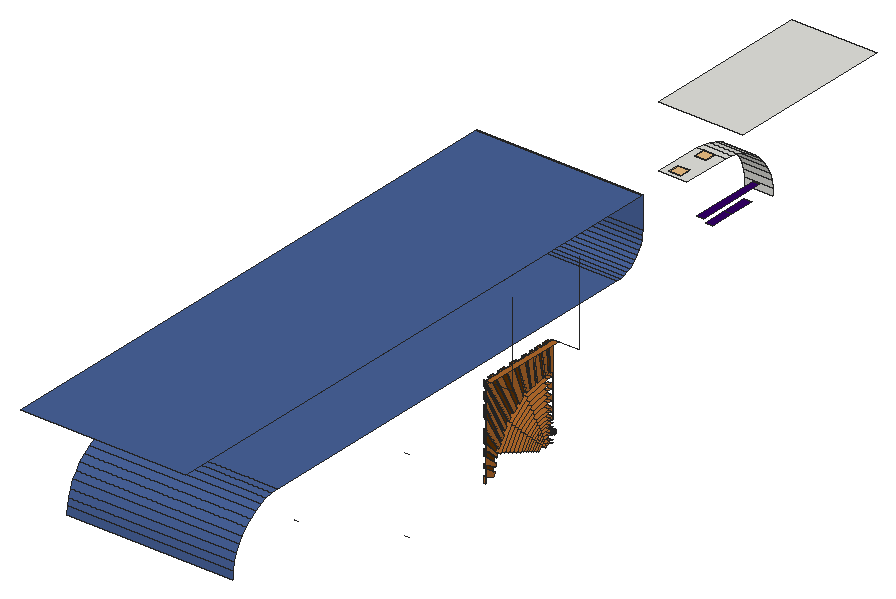
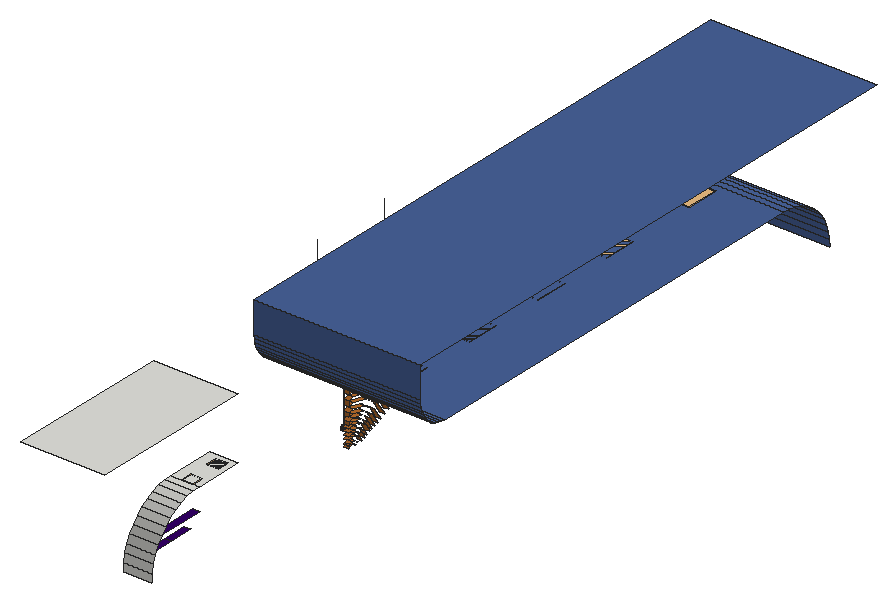
# SketchUp Ruby script. Lengths in inches.
U = 1.inch
M = Sketchup.active_model
def pt(a) = Geom::Point3d.new(a.map { |v| v * U })
def face(e, loops, mat)
  f = e.add_face(loops[0].map { |a| pt(a) })
  loops[1..].each { |l| e.add_face(l.map { |a| pt(a) }).erase! }
  f.material = f.back_material = mat if mat
  f
end
# faces: each face lists its corners as indices into pts; further lists are holes
def faces(e, pts, list, mat = nil) = list.each { |f| face(e, (f[0].is_a?(Array) ? f : [f]).map { |l| l.map { |i| pts[i] } }, mat) }
# xy, xz, yz: faces in a plane at the given z, y or x. An outline is a flat list of corners, or four numbers for a rectangle; further outlines are holes
def ring(l) = l.size == 4 ? [[l[0], l[1]], [l[2], l[1]], [l[2], l[3]], [l[0], l[3]]] : l.each_slice(2).to_a
def flat(e, list, mat, &to3) = list.each { |f| face(e, (f[0].is_a?(Array) ? f : [f]).map { |l| ring(l).map { |u, v| to3.(u, v) } }, mat) }
def xy(e, z, list, mat = nil) = flat(e, list, mat) { |x, y| [x, y, z] }
def xz(e, y, list, mat = nil) = flat(e, list, mat) { |x, z| [x, y, z] }
def yz(e, x, list, mat = nil) = flat(e, list, mat) { |y, z| [x, y, z] }
def lines(e, pts, list) = list.each { |a, b| e.add_line(pt(pts[a]), pt(pts[b])) }
# prism: a flat outline (further loops are holes) pulled along v
def prism(e, loops, v, mat = nil)
  f = face(e, loops, mat); d = Geom::Vector3d.new(v.map { |x| x * U })
  f.pushpull(f.normal.samedirection?(d) ? d.length : -d.length)
end
def box(e, o, s, mat = nil) = prism(e, [[o, [o[0] + s[0], o[1], o[2]], [o[0] + s[0], o[1] + s[1], o[2]], [o[0], o[1] + s[1], o[2]]]], [0, 0, s[2]], mat)
def at(x, y, z, deg = 0) = Geom::Transformation.translation(pt([x, y, z])) * Geom::Transformation.rotation(ORIGIN, Z_AXIS, deg.degrees)
def axes(o, x, y, z) = Geom::Transformation.new([*x, 0, *y, 0, *z, 0, *pt(o).to_a, 1])
def part(name) = M.definitions.add(name)
# library, detail: a bought-in or finely detailed component or shape, given as its bounding box
def library(name, o, s) = part(name).tap { |d| box(d.entities, o, s) }
def detail(e, o, s) = box(e.add_group.entities, o, s)
def put(e, d, t, mat = nil) = e.add_instance(d, t).tap { |i| i.material = mat if mat }
def group(e, t, mat = nil) = e.add_group.tap { |g| g.transformation = t; g.material = mat if mat }.entities
root = M.entities
M.materials.add("[Color C08]").color = [102, 51, 0]
M.materials.add("[Color J08]").color = [51, 0, 102]
M.materials.add("[Formica Blue]").color = [71, 97, 152]
M.materials.add("[Wood Bamboo]").color = [177, 105, 43]
c1 = part("Recessed light")
detail(c1.entities,[0,0,0],[14.08,14.08,3])
c2 = part("Recessed light \#1")
detail(c2.entities,[0,0,0],[4.875,4.875,1.1875])
xy(root,196.65,[[182,311.38,185,321.81],[182,321.81,185,332.23]],"[Color J08]")
xy(root,201.38,[[182,306.65,185,336.96]],"[Color J08]")
xy(root,209.98,[[205.625,165.13,206.625,167.88],[205.625,170.69,206.625,173.92],[205.625,177.27,206.625,180.4],[205.625,183.39,206.625,185.625],[205.625,187.86,206.625,189.13],
  [205.625,190.73,206.625,192.46],[205.625,192.46,206.625,193.08],[205.625,195.09,206.625,196.125],[205.625,196.125,206.625,197.55]],"[Wood Bamboo]")
xy(root,210,[[206.625,162.98,209,198.98]],"[Wood Bamboo]")
xy(root,219.12,[[137.625,49.45,208.5625,230.99]],"[Formica Blue]")
xy(root,219.28,[[173,297.87,185,318.3125]])
xy(root,246,[[173,297.87,209,369.14]])
xy(root,246,[[137.625,0.14,208.5625,244.43]],"[Formica Blue]")
xz(root,163,[[205.625,170.21,206.625,173.125],[205.625,176.04,206.625,177.78],[205.625,180.75,206.625,183.41],[205.625,185.93,206.625,191.12],[205.625,195.86,206.625,200.46],
  [205.625,202.96,206.625,205.25],[205.625,207.6,206.625,209.97]],"[Wood Bamboo]")
xz(root,198.97,[[204.625,179.23,206.625,180.69],[204.625,182.32,206.625,184.08],[204.625,186.37,206.625,188.67],[204.625,190.87,206.625,193.18],[204.625,195.77,206.625,197.62]],"[Wood Bamboo]")
xz(root,244.43,[[137.625,232.56,208.5625,246]],"[Formica Blue]")
yz(root,205.625,[[167.88,172.94,163,176.04,163,177.78,168.17,174.44],[168.49,176.05,163,180.75,163,183.41,168.83,177.79],[169.125,179.3125,163,185.93,163,191.12,170.04,180.72],[170.96,182.13,163,195.86,163,200.46,171.63,183.15],[172.58,184.61,163,202.96,163,205.25,173.46,185.97],
  [174.375,187.37,163,207.6,163,209.97,175.42,188.97],[176.54,189.75,165.13,209.98,167.88,209.98,178.08,190.8125],[179.64,191.9,170.69,209.98,173.92,209.98,181.39,193.12],[183.14,194.33,177.27,209.98,180.4,209.98,184.88,195.55],[186.57,195.93,183.39,209.98,185.625,209.98,187.86,196.22],
  [189.29,196.54,187.86,209.98,189.13,209.98,191.14,196.96,190.73,196.87],[193.12,197.41,190.73,209.98,193.08,209.98,195.09,197.86,193.65,197.53],[197.98,197.78,197.55,197.86,196.125,198.09,195.09,209.98,197.55,209.98]],"[Color C08]")
yz(root,206.625,[[163,170.21,162.98,170.22,162.98,176.05,163,176.04],[167.48,170.9,163,173.125,163,176.04,167.88,172.94],[168.17,174.44,163,177.78,163,180.75,168.49,176.05],[163,176.04,162.98,176.05,162.98,177.79,163,177.78],[163,177.78,162.98,177.79,162.98,180.77,163,180.75],
  [168.83,177.79,163,183.41,163,185.93,169.125,179.3125],[198.97,179.23,198.97,180.69,198.98,180.6875,198.98,179.23],[198.98,180.6875,198.97,180.69,198.97,182.32,198.98,182.32],[170.04,180.72,163,191.12,163,195.86,170.96,182.13],[163,180.75,162.98,180.77,162.98,183.42,163,183.41],
  [198.97,182.32,198.98,184.08],[171.63,183.15,163,200.46,163,202.96,172.58,184.61],[163,183.41,162.98,183.42,162.98,210,163,209.97],[198.97,184.08,198.98,186.37],[173.46,185.97,163,205.25,163,207.6,174.375,187.37],
  [198.97,186.37,198.97,188.67,198.98,188.66,198.98,186.37],[198.98,188.66,198.97,188.67,198.97,190.87,198.98,190.86],[175.42,188.97,163,209.97,163,209.98,165.13,209.98,176.54,189.75],[178.08,190.8125,167.88,209.98,170.69,209.98,179.64,191.9],[198.98,190.86,198.97,190.87,198.97,193.18,198.98,193.18],
  [181.39,193.12,173.92,209.98,177.27,209.98,183.14,194.33],[198.97,193.18,198.98,195.77],[184.88,195.55,180.4,209.98,183.39,209.98,186.57,195.93],[198.97,195.77,198.98,197.62],[187.86,196.22,185.625,209.98,187.86,209.98,189.29,196.54],
  [191.14,196.96,189.13,209.98,190.73,209.98,193.12,197.41,192.46,197.26,191.56,197.06],[198.97,197.62,197.98,197.78,197.55,209.98,198.97,209.98],[198.97,197.62,198.98,199.86],[195.09,197.86,193.08,209.98,195.09,209.98,196.125,198.09],[198.97,199.86,198.97,209.98,197.55,209.98,197.55,210,198.98,210,198.98,199.86],
  [163,209.97,162.98,210,187.85,210,187.86,209.98,163,209.98],[187.86,209.98,187.85,210,189.125,210,189.13,209.98],[189.13,209.98,189.125,210,190.72,210,190.73,209.98],[190.73,209.98,190.72,210,192.46,210,192.46,209.98],[192.46,209.98,195.09,210],
  [195.09,209.98,196.125,210],[196.125,209.98,197.55,210]],"[Wood Bamboo]")
p = [[206.625,195.85,170.66],[206.625,194.93,170.03],[204.625,194.93,170.03],[204.625,195.85,170.66],[206.625,198.98,170.15],[206.625,198.03,170.73],
  [204.625,198.03,170.73],[204.625,198.98,170.15],[206.625,192.8,172.09],[206.625,191.57,170.21],[204.625,191.57,170.21],[204.625,192.8,172.09],
  [206.625,190.3,170.73],[206.625,191.8125,173.05],[204.625,191.8125,173.05],[204.625,190.3,170.73],[206.625,196.93,170.91],[204.625,196.93,170.91],
  [206.625,194.14,170.79],[206.625,195.4,171.67],[204.625,195.4,171.67],[204.625,194.14,170.79],[206.625,163,173.125],[206.625,167.48,170.9],
  [205.625,167.48,170.9],[205.625,163,173.125],[206.625,190.77,174.07],[206.625,188.94,171.27],[204.625,188.94,171.27],[204.625,190.77,174.07],
  [206.625,198.42,171.76],[206.625,198.98,171.41],[204.625,198.98,171.41],[204.625,198.42,171.76],[206.625,196.9,172.01],[204.625,196.9,172.01],
  [206.625,187.43,171.89],[206.625,189.59,175.21],[204.625,189.59,175.21],[204.625,187.43,171.89],[206.625,194.65,173.38],[204.625,194.65,173.38],
  [206.625,188.6875,176.09],[206.625,186.26,172.36],[204.625,186.26,172.36],[204.625,188.6875,176.09],[206.625,167.88,172.94],[206.625,163,176.04],
  [205.625,163,176.04],[205.625,167.88,172.94],[206.625,184.9,172.92],[206.625,187.63,177.11],[204.625,187.63,177.11],[204.625,184.9,172.92],
  [206.625,194.09,174.64],[204.625,194.09,174.64],[206.625,196.84,173.875],[204.625,196.84,173.875],[206.625,186.46,178.25],[206.625,183.38,173.53],
  [204.625,183.38,173.53],[204.625,186.46,178.25],[206.625,198.98,173.52],[204.625,198.98,173.52],[206.625,193.51,175.97],[204.625,193.51,175.97],
  [206.625,181.74,174.2],[206.625,185.19,179.48],[204.625,185.19,179.48],[204.625,181.74,174.2],[206.625,163,177.78],[206.625,168.17,174.44],
  [205.625,168.17,174.44],[205.625,163,177.78],[206.625,196.8,175.25],[204.625,196.8,175.25],[206.625,198.98,174.89],[204.625,198.98,174.89],
  [206.625,183.54,181.09],[206.625,179.6,175.0625],[204.625,179.6,175.0625],[204.625,183.54,181.09],[206.625,192.85,177.47],[204.625,192.85,177.47],
  [206.625,177.47,175.93],[206.625,181.88,182.7],[204.625,181.88,182.7],[204.625,177.47,175.93],[206.625,168.49,176.05],[206.625,163,180.75],
  [205.625,163,180.75],[205.625,168.49,176.05],[206.625,196.76,176.71],[204.625,196.76,176.71],[206.625,192.34,178.63],[204.625,192.34,178.63],
  [206.625,198.98,176.35],[204.625,198.98,176.35],[206.625,180.29,184.24],[206.625,175.42,176.76],[204.625,175.42,176.76],[204.625,180.29,184.24],
  [206.625,191.75,179.97],[204.625,191.75,179.97],[206.625,196.71,178.34],[204.625,196.71,178.34],[206.625,173.26,177.64],[206.625,178.62,185.86],
  [204.625,178.62,185.86],[204.625,173.26,177.64],[206.625,163,183.41],[206.625,168.83,177.79],[205.625,168.83,177.79],[205.625,163,183.41],
  [206.625,198.98,177.97],[204.625,198.98,177.97],[206.625,191.08,181.47],[204.625,191.08,181.47],[206.625,176.76,187.67],[206.625,170.85,178.61],
  [204.625,170.85,178.61],[204.625,176.76,187.67],[206.625,196.67,179.61],[204.625,196.67,179.61],[206.625,198.97,179.23],[204.625,198.97,179.23],
  [206.625,169.125,179.3125],[206.625,163,185.93],[205.625,163,185.93],[205.625,169.125,179.3125],[204.625,169.125,179.3125],[205.625,170.04,180.72],
  [206.625,170.04,180.72],[206.625,170.96,182.13],[205.625,170.96,182.13],[205.625,171.63,183.15],[206.625,171.63,183.15],[206.625,172.58,184.61],
  [205.625,172.58,184.61],[205.625,173.46,185.97],[206.625,173.46,185.97],[206.625,174.375,187.37],[205.625,174.375,187.37],[205.625,175.42,188.97],
  [204.625,175.42,188.97],[206.625,190.375,183.09],[204.625,190.375,183.09],[206.625,196.63,181.08],[204.625,196.63,181.08],[206.625,163,191.12],
  [205.625,163,191.12],[206.625,198.97,180.69],[204.625,198.97,180.69],[206.625,189.44,185.2],[204.625,189.44,185.2],[206.625,196.58,182.71],
  [204.625,196.58,182.71],[206.625,163,195.86],[205.625,163,195.86],[206.625,198.97,182.32],[204.625,198.97,182.32],[206.625,188.51,187.31],
  [204.625,188.51,187.31],[206.625,196.53,184.48],[204.625,196.53,184.48],[206.625,163,200.46],[205.625,163,200.46],[206.625,198.97,184.08],
  [204.625,198.97,184.08],[206.625,187.62,189.33],[204.625,187.62,189.33],[206.625,163,202.96],[205.625,163,202.96],[206.625,196.46,186.78],
  [204.625,196.46,186.78],[206.625,186.68,191.46],[204.625,186.68,191.46],[206.625,163,205.25],[205.625,163,205.25],[206.625,198.97,186.37],
  [204.625,198.97,186.37],[206.625,196.39,189.09],[204.625,196.39,189.09],[206.625,163,207.6],[205.625,163,207.6],[206.625,185.63,193.84],
  [204.625,185.63,193.84],[206.625,198.97,188.67],[204.625,198.97,188.67],[206.625,163,209.97],[206.625,175.42,188.97],[205.625,163,209.97],
  [206.625,176.54,189.75],[205.625,176.54,189.75],[205.625,178.08,190.8125],[206.625,178.08,190.8125],[206.625,179.64,191.9],[205.625,179.64,191.9],
  [205.625,181.39,193.12],[206.625,181.39,193.12],[206.625,183.14,194.33],[205.625,183.14,194.33],[205.625,184.88,195.55],[204.625,184.88,195.55],
  [206.625,196.33,191.3],[204.625,196.33,191.3],[206.625,165.13,209.98],[205.625,165.13,209.98],[206.625,167.88,209.98],[205.625,167.88,209.98],
  [206.625,198.97,190.87],[204.625,198.97,190.87],[206.625,196.26,193.63],[204.625,196.26,193.63],[206.625,170.69,209.98],[205.625,170.69,209.98],
  [206.625,173.92,209.98],[205.625,173.92,209.98],[206.625,198.97,193.18],[204.625,198.97,193.18],[185,343.92,193.67],[185,343.7,197.02],
  [173,343.7,197.02],[173,343.92,193.67],[206.625,196.18,196.23],[204.625,196.18,196.23],[206.625,177.27,209.98],[205.625,177.27,209.98],
  [137.625,25.13,194.81],[137.625,25.34,197.98],[208.5625,25.34,197.98],[208.5625,25.13,194.81],[206.625,180.4,209.98],[206.625,184.88,195.55],
  [205.625,180.4,209.98],[206.625,186.57,195.93],[205.625,186.57,195.93],[205.625,187.86,196.22],[206.625,187.86,196.22],[206.625,189.29,196.54],
  [205.625,189.29,196.54],[205.625,190.73,196.87],[205.625,191.14,196.96],[206.625,191.14,196.96],[206.625,191.56,197.06],[206.625,192.46,197.26],
  [206.625,193.12,197.41],[205.625,193.12,197.41],[205.625,193.65,197.53],[205.625,195.09,197.86],[206.625,195.09,197.86],[206.625,196.125,198.09],
  [205.625,196.125,198.09],[204.625,196.125,198.09],[206.625,198.97,195.77],[204.625,198.97,195.77],[206.625,183.39,209.98],[205.625,183.39,209.98],
  [206.625,185.625,209.98],[205.625,185.625,209.98],[206.625,187.86,209.98],[205.625,187.86,209.98],[206.625,189.13,209.98],[205.625,189.13,209.98],
  [185,343.05,200.3],[173,343.05,200.3],[206.625,190.73,209.98],[205.625,190.73,209.98],[205.625,197.55,197.86],[205.625,197.98,197.78],
  [206.625,197.98,197.78],[206.625,198.97,197.62],[204.625,198.97,197.62],[206.625,197.55,209.98],[205.625,197.55,209.98],[206.625,193.08,209.98],
  [205.625,193.08,209.98],[137.625,25.96,201.1],[208.5625,25.96,201.1],[206.625,195.09,209.98],[205.625,195.09,209.98],[185,341.97,203.47],
  [173,341.97,203.47],[137.625,26.98,204.11],[208.5625,26.98,204.11],[185,340.49,206.48],[173,340.49,206.48],[137.625,28.39,206.96],
  [208.5625,28.39,206.96],[185,338.63,209.26],[173,338.63,209.26],[137.625,30.16,209.61],[208.5625,30.16,209.61],[185,336.42,211.78],
  [173,336.42,211.78],[137.625,32.25,212],[208.5625,32.25,212],[185,333.9,213.99],[173,333.9,213.99],[137.625,34.64,214.1],
  [208.5625,34.64,214.1],[185,331.12,215.85],[173,331.12,215.85],[137.625,37.29,215.86],[208.5625,37.29,215.86],[185,328.11,217.33],
  [173,328.11,217.33],[137.625,40.14,217.27],[208.5625,40.14,217.27],[137.625,43.15,218.29],[208.5625,43.15,218.29],[185,324.94,218.41],
  [173,324.94,218.41],[137.625,46.27,218.91],[208.5625,46.27,218.91],[185,321.66,219.0625],[173,321.66,219.0625],[137.625,49.45,219.12],
  [208.5625,49.45,219.12],[137.625,230.99,219.12],[137.625,232.75,219.24],[208.5625,232.75,219.24],[208.5625,230.99,219.12],[185,318.3125,219.28],
  [173,318.3125,219.28],[137.625,234.47,219.58],[208.5625,234.47,219.58],[137.625,236.14,220.14],[208.5625,236.14,220.14],[137.625,237.71,220.92],
  [208.5625,237.71,220.92],[137.625,239.18,221.9],[208.5625,239.18,221.9],[137.625,240.5,223.06],[208.5625,240.5,223.06],[137.625,241.66,224.38],
  [208.5625,241.66,224.38],[137.625,242.63,225.84],[208.5625,242.63,225.84],[137.625,243.41,227.42],[208.5625,243.41,227.42],[137.625,243.98,229.08],
  [208.5625,243.98,229.08],[137.625,244.32,230.81],[208.5625,244.32,230.81],[137.625,244.43,232.56],[208.5625,244.43,232.56],[209,198.98,210],
  [218,198.98,210],[218,198.98,246],[209,162.98,210],[218,162.98,210],[218,162.98,246],[209,59.99,170.08],
  [207,59.99,170.08],[209,59.99,201.92],[207,59.99,201.92],[209,118.89,170.08],[207,118.89,170.08],[209,118.89,201.92],
  [207,118.89,201.92],[209,196.54,177.09],[206.625,196.54,177.09],[209,196.76,177.18],[206.625,196.76,177.18],[209,197.03,177.22],
  [206.625,197.03,177.22],[209,197.31,177.18],[206.625,197.31,177.18],[209,197.5625,177.07],[206.625,197.5625,177.07],[209,197.78,176.91],
  [206.625,197.78,176.91],[209,197.95,176.6875],[206.625,197.95,176.6875],[209,198.06,176.43],[206.625,198.06,176.43],[209,198.1,176.15],
  [206.625,198.1,176.15],[209,198.06,175.88],[206.625,198.06,175.88],[209,197.95,175.625],[206.625,197.95,175.625],[209,197.78,175.4],
  [206.625,197.78,175.4],[209,197.5625,175.23],[206.625,197.5625,175.23],[209,197.31,175.13],[206.625,197.31,175.13],[209,197.03,175.09],
  [206.625,197.03,175.09],[209,196.76,175.13],[206.625,196.76,175.13],[209,196.54,175.22],[206.625,196.54,175.22],[209,190.72,175.22],
  [206.625,190.72,175.22],[209,190.72,177.09],[206.625,190.72,177.09],[206.625,198.98,179.23],[206.625,199.1875,179.2],[206.625,198.98,180.6875],
  [206.625,199.2,180.65],[206.625,198.98,182.32],[206.625,199.23,182.28],[206.625,198.98,184.08],[206.625,199.25,184.03],[206.625,198.98,186.37],
  [206.625,199.33,186.3125],[206.625,198.98,188.66],[206.625,199.33,188.61],[206.625,198.98,190.86],[206.625,199.32,190.81],[206.625,198.98,193.18],
  [206.625,199.34,193.12],[206.625,198.98,195.77],[206.625,199.38,195.7],[206.625,198.98,199.86],[206.625,199.33,199.8],[206.625,198.98,197.62],
  [206.625,199.26,197.57],[206.625,190.73,196.87],[206.625,193.65,197.53],[206.625,197.55,197.86]]
faces(root,p,[[0,1,2,3],[4,5,6,7],[8,9,10,11],[12,13,14,15],[16,0,3,17],[5,16,17,6],[18,19,20,21],[22,23,24,25],
  [26,27,28,29],[30,31,32,33],[19,34,35,20],[34,30,33,35],[36,37,38,39],[40,8,11,41],[42,43,44,45],[46,47,48,49],
  [50,51,52,53],[13,54,55,14],[56,40,41,57],[58,59,60,61],[62,56,57,63],[64,26,29,65],[66,67,68,69],[70,71,72,73],
  [54,74,75,55],[74,76,77,75],[78,79,80,81],[37,82,83,38],[84,85,86,87],[88,89,90,91],[92,64,65,93],[94,42,45,95],
  [96,92,93,97],[98,99,100,101],[51,102,103,52],[82,104,105,83],[106,107,108,109],[110,111,112,113],[104,114,115,105],[116,58,61,117],
  [118,119,120,121],[122,94,95,123],[124,122,123,125],[126,127,128,129],[130,129,131,132,133,134,135,136,137,138,139,140,141,142,143,144],[67,145,146,68],[102,147,148,103],[149,132,131,150],
  [147,151,152,148],[153,78,81,154],[155,116,117,156],[133,157,158,134],[159,155,156,160],[85,161,162,86],[145,163,164,146],[165,136,135,166],
  [163,167,168,164],[169,98,101,170],[137,171,172,138],[173,153,154,174],[107,175,176,108],[177,140,139,178],[179,173,174,180],[161,181,182,162],
  [141,183,184,142],[185,118,121,186],[181,187,188,182],[189,190,143,191],[190,192,193,194,195,196,197,198,199,200,201,202,203,144,143],[204,169,170,205],[192,206,207,193],[208,195,194,209],
  [210,204,205,211],[175,212,213,176],[196,214,215,197],[216,199,198,217],[212,218,219,213],[224,185,186,225],[200,226,227,201],[232,233,202,234],
  [233,235,236,237,238,239,240,241,242,243,244,245,246,247,248,249,250,251,252,253,203,202],[254,224,225,255],[235,256,257,236],[258,238,237,259],[239,260,261,240],[262,243,242,263],[246,266,267,247],[253,252,268,269,270,271,272],
  [273,270,269,274],[275,250,249,276],[251,279,280,252]],"[Wood Bamboo]")
faces(root,p,[[220,221,222,223],[221,264,265,222],[264,281,282,265],[281,285,286,282],[285,289,290,286],[289,293,294,290],[293,297,298,294],[297,301,302,298],
  [301,305,306,302],[305,311,312,306],[311,315,316,312],[315,323,324,316]])
faces(root,p,[[228,229,230,231],[229,277,278,230],[277,283,284,278],[283,287,288,284],[287,291,292,288],[291,295,296,292],[295,299,300,296],[299,303,304,300],
  [303,307,308,304],[307,309,310,308],[309,313,314,310],[313,317,318,314],[319,320,321,322],[320,325,326,321],[325,327,328,326],[327,329,330,328],
  [329,331,332,330],[331,333,334,332],[333,335,336,334],[335,337,338,336],[337,339,340,338],[339,341,342,340],[341,343,344,342],[343,345,346,344]],"[Formica Blue]")
lines(root,p,[[347,348],[348,349],[350,351],[351,352],[353,354],[355,356],[357,358],[359,360],[361,362],[363,364],[365,366],[367,368],
  [369,370],[371,372],[373,374],[375,376],[377,378],[379,380],[381,382],[383,384],[385,386],[387,388],[389,390],[391,392],
  [393,394],[395,396],[397,398],[399,400],[401,402],[403,404],[405,406],[407,408],[409,410],[411,412],[413,414],[415,416],
  [417,418],[419,420],[421,241],[422,248],[423,268]])
put(root,c1,axes([178.45,207.23,219.12],[-1,0,0],[0,1,0],[0,0,-1]))
put(root,c1,axes([178.45,52.85,219.12],[-1,0,0],[0,1,0],[0,0,-1]))
put(root,c1,axes([178.45,207.23,219.12],[-1,0,0],[0,1,0],[0,0,-1]))
put(root,c1,axes([178.45,170.46,219.12],[-1,0,0],[0,1,0],[0,0,-1]))
put(root,c1,axes([178.45,133.68,219.12],[-1,0,0],[0,1,0],[0,0,-1]))
put(root,c1,axes([178.45,96.91,219.12],[-1,0,0],[0,1,0],[0,0,-1]))
put(root,c2,axes([180.47,299.98,219.28],[-1,0,0],[0,1,0],[0,0,-1]))
put(root,c2,axes([180.47,313.52,219.28],[-1,0,0],[0,1,0],[0,0,-1]))
